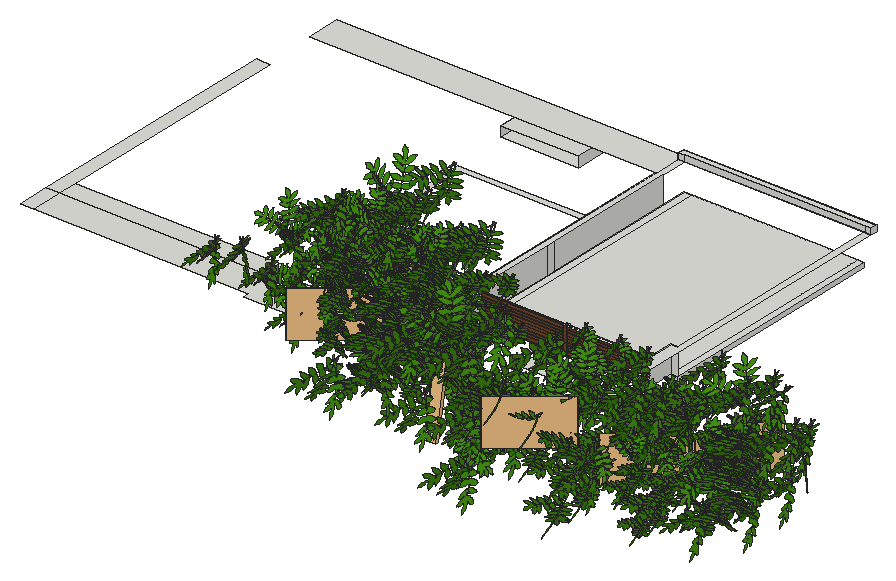
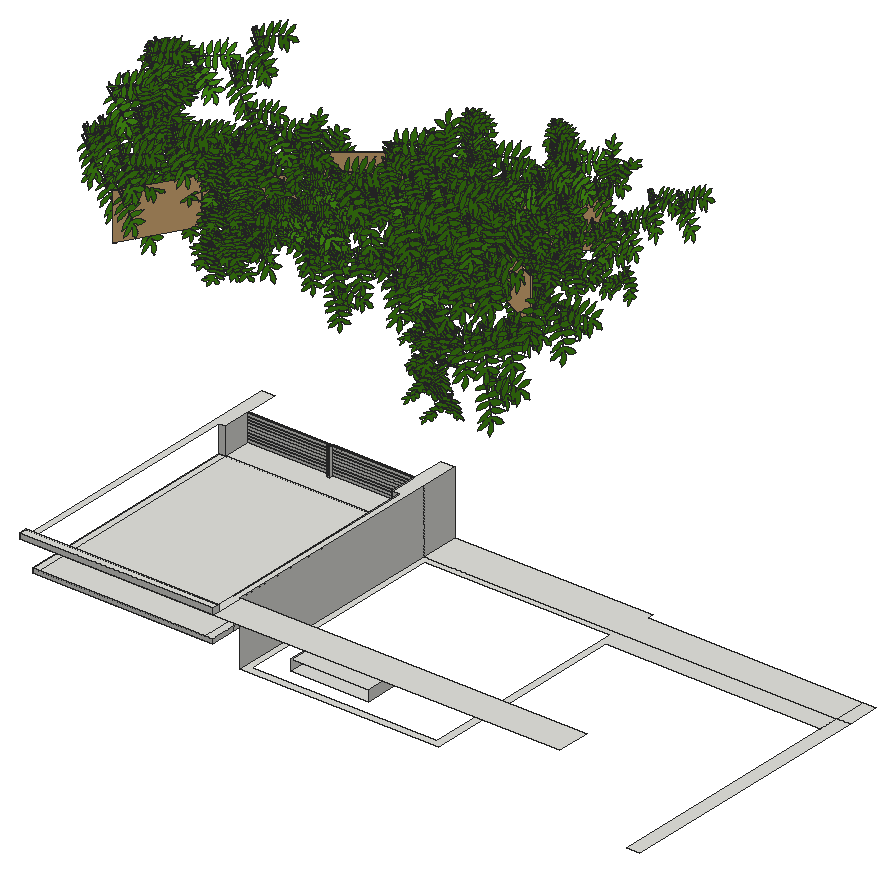
# SketchUp Ruby script. Lengths in inches.
U = 1.inch
M = Sketchup.active_model
def pt(a) = Geom::Point3d.new(a.map { |v| v * U })
def face(e, loops, mat)
  f = e.add_face(loops[0].map { |a| pt(a) })
  loops[1..].each { |l| e.add_face(l.map { |a| pt(a) }).erase! }
  f.material = f.back_material = mat if mat
  f
end
# faces: each face lists its corners as indices into pts; further lists are holes
def faces(e, pts, list, mat = nil) = list.each { |f| face(e, (f[0].is_a?(Array) ? f : [f]).map { |l| l.map { |i| pts[i] } }, mat) }
# xy, xz, yz: faces in a plane at the given z, y or x. An outline is a flat list of corners, or four numbers for a rectangle; further outlines are holes
def ring(l) = l.size == 4 ? [[l[0], l[1]], [l[2], l[1]], [l[2], l[3]], [l[0], l[3]]] : l.each_slice(2).to_a
def flat(e, list, mat, &to3) = list.each { |f| face(e, (f[0].is_a?(Array) ? f : [f]).map { |l| ring(l).map { |u, v| to3.(u, v) } }, mat) }
def xy(e, z, list, mat = nil) = flat(e, list, mat) { |x, y| [x, y, z] }
def xz(e, y, list, mat = nil) = flat(e, list, mat) { |x, z| [x, y, z] }
def yz(e, x, list, mat = nil) = flat(e, list, mat) { |y, z| [x, y, z] }
def lines(e, pts, list) = list.each { |a, b| e.add_line(pt(pts[a]), pt(pts[b])) }
# prism: a flat outline (further loops are holes) pulled along v
def prism(e, loops, v, mat = nil)
  f = face(e, loops, mat); d = Geom::Vector3d.new(v.map { |x| x * U })
  f.pushpull(f.normal.samedirection?(d) ? d.length : -d.length)
end
def box(e, o, s, mat = nil) = prism(e, [[o, [o[0] + s[0], o[1], o[2]], [o[0] + s[0], o[1] + s[1], o[2]], [o[0], o[1] + s[1], o[2]]]], [0, 0, s[2]], mat)
def at(x, y, z, deg = 0) = Geom::Transformation.translation(pt([x, y, z])) * Geom::Transformation.rotation(ORIGIN, Z_AXIS, deg.degrees)
def axes(o, x, y, z) = Geom::Transformation.new([*x, 0, *y, 0, *z, 0, *pt(o).to_a, 1])
def part(name) = M.definitions.add(name)
# library, detail: a bought-in or finely detailed component or shape, given as its bounding box
def library(name, o, s) = part(name).tap { |d| box(d.entities, o, s) }
def detail(e, o, s) = box(e.add_group.entities, o, s)
def put(e, d, t, mat = nil) = e.add_instance(d, t).tap { |i| i.material = mat if mat }
def group(e, t, mat = nil) = e.add_group.tap { |g| g.transformation = t; g.material = mat if mat }.entities
root = M.entities
M.materials.add("[Color D01]").color = [255, 242, 204]
M.materials.add("[Wood Veneer 01]").color = [120, 70, 37]
M.materials.add("hojas").color = [70, 150, 19]
c1 = part("rama-acacia")
p = [[-13.53,0.69,-1.07],[-13.38,0.86,-0.98],[-13.61,0.85,-1.06],[-14.07,0.85,-1.21],[-15.17,0.86,-1.58],[-15.95,0.92,-1.83],
  [-16.01,1,-1.83],[-16.01,1.17,-1.78],[-16.07,1.93,-1.6],[-16.4,2.73,-1.5],[-16.65,3.06,-1.5],[-17.13,4.01,-1.41],
  [-17.78,4.7,-1.44],[-18.28,5.07,-1.51],[-18.57,5.18,-1.58],[-18.91,5.47,-1.62],[-19.07,5.48,-1.67],[-19.35,5.61,-1.73],
  [-19.51,5.64,-1.78],[-19.38,5.57,-1.75],[-19.33,5.5,-1.75],[-19.31,5.23,-1.82],[-19.38,5.08,-1.89],[-19.41,4.84,-1.96],
  [-19.36,4.59,-2.01],[-19.43,4.55,-2.04],[-19.36,4.15,-2.125],[-19.21,3.7,-2.19],[-18.875,3.1,-2.24],[-18.61,2.78,-2.24],
  [-17.83,2.19,-2.13],[-17.4375,1.85,-2.09],[-17.04,1.49,-2.05],[-16.61,1.24,-1.97],[-16.17,1.0625,-1.87],[-16.06,0.95,-1.86],
  [-16.06,0.91,-1.87],[-16.32,0.9,-1.96],[-16.7,0.88,-2.1],[-17.05,0.91,-2.21],[-17.61,1.15,-2.33],[-18.06,1.29,-2.45],
  [-18.88,1.53,-2.67],[-20.25,1.46,-3.15],[-20.59,1.49,-3.26],[-20.79,1.37,-3.36],[-21.08,1.2,-3.5],[-21.28,1.22,-3.5625],
  [-21.48,0.94,-3.71],[-21.79,0.5,-3.93],[-22.02,0.17,-4.1],[-22.11,0.05,-4.16],[-22.21,-0.02,-4.21],[-22.375,-0.05,-4.28],
  [-22.375,-0.07,-4.28],[-22.18,-0.09,-4.22],[-22.11,-0.07,-4.19],[-21.78,-0.1,-4.09],[-21.6,-0.18,-4.05],[-21.52,-0.27,-4.04],
  [-21.33,-0.33,-4],[-20.94,-0.54,-3.92],[-20.6875,-0.63,-3.86],[-20.54,-0.68,-3.82],[-20.42,-0.67,-3.78],[-20.09,-0.46,-3.61],
  [-19.8,-0.24,-3.45],[-19.21,-0.02,-3.19],[-18.48,0.08,-2.92],[-17.72,0.38,-2.58],[-17.4,0.5,-2.4375],[-16.93,0.75,-2.21],
  [-16.78,0.8,-2.15],[-16.1,0.83,-1.91],[-16.0625,0.81,-1.9],[-16.08,0.77,-1.91],[-16.27,0.72,-1.99],[-16.88,0.39,-2.29],
  [-17.1875,0.15,-2.46],[-17.27,0.02,-2.52],[-17.94,-0.52,-2.89],[-17.94,-0.59,-2.91],[-18.08,-0.68,-2.99],[-18.13,-0.86,-3.05],
  [-18.56,-1.55,-3.38],[-18.71,-2.11,-3.58],[-18.79,-2.61,-3.74],[-18.86,-2.84,-3.83],[-18.87,-3.07,-3.89],[-18.84,-3.22,-3.92],
  [-18.8,-3.26,-3.92],[-18.76,-3.47,-3.96],[-18.76,-3.6,-4],[-18.67,-3.8,-4.02],[-18.61,-3.92,-4.04],[-18.58,-4.11,-4.07],
  [-18.53,-4.18,-4.08],[-18.58,-4.35,-4.14],[-18.65,-4.43,-4.18],[-18.72,-4.51,-4.23],[-18.8125,-4.51,-4.26],[-18.8125,-4.53,-4.26],
  [-18.72,-4.54,-4.24],[-18.66,-4.49,-4.21],[-18.58,-4.43,-4.16],[-18.35,-4.23,-4.03],[-18.32,-4.17,-4],[-18.22,-4.125,-3.95],
  [-18.1,-4,-3.88],[-17.79,-3.72,-3.7],[-17.68,-3.51,-3.61],[-17.32,-3.13,-3.38],[-17.24,-2.94,-3.31],[-16.78,-2.12,-2.93],
  [-16.48,-1.78,-2.73],[-16.3,-1.28,-2.54],[-16.05,-0.75,-2.3125],[-15.89,-0.2,-2.11],[-15.89,0.39,-1.95],[-15.96,0.79,-1.87],
  [-15.91,0.82,-1.84],[-15.27,0.8,-1.63],[-14.18,0.76,-1.27],[-13.78,0.73,-1.15],[-13.78,0.67,-1.16],[-14.23,0.54,-1.35],
  [-14.65,0.33,-1.55],[-14.97,0.02,-1.74],[-15.25,-0.36,-1.9375],[-15.57,-0.72,-2.14],[-15.96,-1.64,-2.52],[-16.2,-2.51,-2.84],
  [-16.2,-3.12,-3],[-16.14,-3.41,-3.06],[-16.1,-3.75,-3.14],[-16.1,-4.09,-3.23],[-16.2,-4.25,-3.3],[-16.2,-4.28,-3.3125],
  [-16.08,-4.19,-3.24],[-15.98,-4.08,-3.18],[-15.96,-3.94,-3.14],[-15.96,-3.8125,-3.1],[-15.9,-3.72,-3.06],[-15.68,-3.55,-2.9375],
  [-15.51,-3.49,-2.86],[-15.3,-3.33,-2.75],[-15.23,-3.17,-2.68],[-15.01,-3.03,-2.57],[-14.875,-2.83,-2.47],[-14.6,-2.59,-2.3125],
  [-14.4,-2.27,-2.16],[-14.12,-1.6,-1.89],[-13.91,-1.1,-1.68],[-13.67,-0.83,-1.53],[-13.53,-0.45,-1.38],[-13.53,0.67,-1.08],
  [-12.41,6.01,0.65],[-12.44,6.14,0.68],[-12.41,6.29,0.73],[-12.43,6.29,0.73],[-12.44,6.26,0.72],[-12.47,6.15,0.68],
  [-12.49,6.07,0.66],[-12.57,5.75,0.55],[-12.67,5.36,0.43],[-12.79,4.875,0.28],[-12.83,4.52,0.18],[-12.83,3.99,0.04],
  [-12.73,3.11,-0.18],[-12.58,2.52,-0.3125],[-12.3,1.97,-0.41],[-11.88,1.51,-0.46],[-11.37,1.0625,-0.48],[-10.75,0.75,-0.45],
  [-10.75,0.68,-0.47],[-12.55,0.7,-0.79],[-13.21,0.79,-0.89],[-13.2,0.67,-0.92],[-12.56,0.62,-0.82],[-11.15,0.56,-0.58],
  [-10.79,0.54,-0.52],[-10.72,0.52,-0.51],[-10.72,0.5,-0.52],[-10.87,0.47,-0.55],[-11.14,0.41,-0.62],[-11.39,0.27,-0.7],
  [-11.625,-0.01,-0.82],[-11.8,-0.43,-0.96],[-11.83,-0.57,-1],[-12.02,-1.08,-1.17],[-12.1,-1.39,-1.27],[-12.17,-1.95,-1.4375],
  [-12.17,-2.77,-1.65],[-12.09,-3.59,-1.86],[-11.86,-4.26,-2],[-11.8125,-4.4,-2.03],[-11.84,-4.49,-2.05],[-11.91,-4.6,-2.1],
  [-11.97,-4.65,-2.12],[-11.98,-4.67,-2.13],[-11.92,-4.65,-2.11],[-11.84,-4.59,-2.08],[-11.77,-4.52,-2.05],[-11.74,-4.47,-2.03],
  [-11.37,-4.3125,-1.92],[-10.95,-4.0625,-1.78],[-10.82,-3.89,-1.71],[-10.64,-3.57,-1.59],[-10.41,-3.05,-1.41],[-10.27,-2.73,-1.3],
  [-10.07,-1.88,-1.03],[-10.15,-0.71,-0.73],[-10.31,-0.1,-0.6],[-10.5,0.4,-0.5],[-10.5,0.48,-0.48],[-10.44,0.53,-0.45],
  [-10.39,0.64,-0.42],[-10.52,0.73,-0.42],[-10.44,0.93,-0.35],[-10.44,1.2,-0.28],[-10.32,1.47,-0.18],[-10.48,2.6875,0.12],
  [-10.43,2.96,0.2],[-10.75,3.87,0.38],[-11.26,4.93,0.57],[-11.8,5.54,0.64],[-12.37,5.93,0.64],[-7.78,0.19,-0.06],
  [-7.78,0.25,-0.04],[-7.75,0.39,0],[-7.89,0.4,-0.02],[-7.96,0.46,-0.02],[-7.96,0.49,-0.01],[-7.76,0.62,0.06],
  [-7.53,0.99,0.2],[-7.31,1.78,0.45],[-7.31,2.74,0.71],[-7.63,3.6875,0.9],[-8.02,4.57,1.07],[-8.66,5.23,1.13],
  [-8.83,5.4,1.14],[-8.92,5.54,1.16],[-9.1,5.64,1.16],[-9.08,5.6,1.15],[-9.02,5.56,1.15],[-8.94,5.46,1.14],
  [-8.9,5.37,1.12],[-8.9375,5.25,1.08],[-9.14,4.92,0.96],[-9.31,4.5625,0.83],[-9.39,3.73,0.6],[-9.44,2.76,0.32],
  [-9.23,1.59,0.05],[-8.82,0.9,-0.06],[-8.36,0.59,-0.0625],[-8.14,0.51,-0.04],[-8.05,0.48,-0.03],[-8.05,0.46,-0.04],
  [-8.12,0.43,-0.06],[-10.1,0.49,-0.4],[-8.22,0.3125,-0.11],[-8.22,0.25,-0.125],[-8.53,0.13,-0.21],[-8.8,-0.16,-0.34],
  [-8.96,-0.61,-0.49],[-8.96,-0.87,-0.56],[-9.16,-1.42,-0.74],[-9.13,-1.77,-0.83],[-9.09,-1.83,-0.84],[-9.125,-1.92,-0.87],
  [-9.125,-2.13,-0.93],[-9.08,-2.23,-0.95],[-9.15,-2.39,-1],[-9.11,-2.67,-1.07],[-9.03,-2.86,-1.11],[-9.07,-3.03,-1.16],
  [-8.97,-3.23,-1.19],[-8.93,-3.44,-1.24],[-8.93,-3.71,-1.32],[-8.79,-4.05,-1.38],[-8.7,-4.25,-1.42],[-8.7,-4.39,-1.46],
  [-8.76,-4.53,-1.5],[-8.77,-4.65,-1.54],[-8.64,-4.55,-1.49],[-8.27,-4.22,-1.33],[-8.1875,-4.06,-1.27],[-8.07,-3.98,-1.23],
  [-7.98,-3.79,-1.17],[-7.79,-3.59,-1.08],[-7.64,-3.3,-0.97],[-7.64,-3.25,-0.96],[-7.59,-3.21,-0.9375],[-7.52,-2.93,-0.85],
  [-7.52,-2.85,-0.83],[-7.47,-2.81,-0.81],[-7.3,-2.09,-0.59],[-7.32,-2.01,-0.57],[-7.27,-1.95,-0.54],[-7.1875,-1.57,-0.42],
  [-7.17,-1.46,-0.39],[-7.17,-1.16,-0.3125],[-7.23,-0.61,-0.17],[-7.49,-0.15,-0.1],[-13.39,-0.07,-1.23],[-13.39,0.25,-1.14],
  [-13.49,0.5625,-1.09],[-13.8,1.01,-1.08],[-13.61,0.91,-1.04],[-13.38,0.92,-0.96],[-13.32,1.03,-0.91],[-13.32,1.35,-0.82],
  [-13.28,1.49,-0.77],[-13.28,1.99,-0.64],[-13.44,2.67,-0.51],[-13.72,3.31,-0.43],[-13.93,3.71,-0.4],[-14.1,4.39,-0.27],
  [-14.5625,5.06,-0.25],[-14.89,5.62,-0.21],[-15.33,6.1,-0.23],[-15.65,6.8,-0.15],[-15.79,6.89,-0.18],[-15.61,6.52,-0.22],
  [-15.51,6.32,-0.24],[-15.45,6.28,-0.23],[-15.52,6,-0.32],[-15.63,5.6875,-0.45],[-15.77,4.97,-0.68],[-15.7,4.25,-0.85],
  [-15.46,3,-1.11],[-15,2.03,-1.21],[-14.3,1.29,-1.17],[-4.5625,0.33,0.09],[-4.22,0.49,0.13],[-4,0.7,0.1875],
  [-3.86,0.99,0.26],[-3.77,1.41,0.38],[-3.7,1.73,0.46],[-3.77,1.99,0.53],[-3.85,2.17,0.58],[-3.88,2.57,0.6875],
  [-3.98,2.9,0.78],[-4.0625,2.97,0.8],[-4.1,3.14,0.84],[-4.1875,3.25,0.87],[-4.27,3.55,0.95],[-4.31,3.71,0.99],
  [-4.42,3.9,1.04],[-4.625,4.2,1.125],[-4.72,4.39,1.18],[-4.89,4.57,1.23],[-4.98,4.73,1.27],[-5,4.72,1.26],
  [-5.01,4.51,1.21],[-4.96,4.32,1.16],[-4.97,4.27,1.14],[-5.14,3.78,1.01],[-5.3,3.39,0.91],[-5.44,2.76,0.74],
  [-5.5,2.09,0.56],[-5.57,1.78,0.48],[-5.57,1.42,0.38],[-5.57,1.09,0.29],[-5.47,0.72,0.19],[-5.22,0.44,0.12],
  [-4.93,0.27,0.07],[-4.76,0.22,0.06],[-4.76,0.18,0.05],[-4.83,0.16,0.04],[-5.26,0,0],[-5.34,-0.04,-0.01],
  [-5.47,-0.22,-0.06],[-5.51,-0.6,-0.16],[-5.42,-1.09,-0.29],[-5.28,-1.49,-0.4],[-5.21,-1.87,-0.5],[-5.11,-2.15,-0.57],
  [-5.08,-2.34,-0.63],[-5.01,-2.47,-0.66],[-4.96,-2.69,-0.72],[-4.86,-2.9375,-0.79],[-4.84,-3.07,-0.82],[-4.77,-3.18,-0.85],
  [-4.74,-3.43,-0.92],[-4.7,-3.71,-0.99],[-4.62,-3.89,-1.04],[-4.58,-3.98,-1.07],[-4.58,-3.83,-1.03],[-4.51,-3.67,-0.98],
  [-4.3,-3.32,-0.89],[-4.16,-3.09,-0.83],[-4.16,-2.98,-0.8],[-4.11,-2.92,-0.78],[-4.02,-2.8,-0.75],[-3.95,-2.59,-0.69],
  [-3.95,-2.33,-0.625],[-3.86,-2.26,-0.6],[-3.86,-2.02,-0.54],[-3.86,-1.44,-0.39],[-3.94,-1.22,-0.33],[-3.94,-1.08,-0.29],
  [-4,-0.96,-0.26],[-4,-0.87,-0.23],[-4.0625,-0.8125,-0.22],[-4.16,-0.54,-0.14],[-4.39,-0.24,-0.06],[-4.61,-0.08,-0.02],
  [-4.77,-0.03,-0.01],[-4.77,-0.01,0],[-4.65,-0.01,0],[-4.61,0.19,0.05],[-4.66,0.23,0.0625],[-4.63,0.29,0.08],
  [-4.07,0.17,0.04],[0,-0.24,-0.06],[0,0,0],[-0.5,0.04,0.01],[-1.58,0.08,0.02],[-13.78,0.67,-1.08]]
faces(c1.entities,p,[[0,1,2,3,4,5,6,7,8,9,10,11,12,13,14,15,16,17,18,19,20,21,22,23,24,25,26,27,28,29,30,31,32,33,34,35,36,37,38,39,40,41,42,43,44,45,46,47,48,49,50,51,52,53,54,55,56,57,58,59,60,61,62,63,64,65,66,67,68,69,70,71,72,73,74,75,76,77,78,79,80,81,82,83,84,85,86,87,88,89,90,91,92,93,94,95,96,97,98,99,100,101,102,103,104,105,106,107,108,109,110,111,112,113,114,115,116,117,118,119,120,121,122,123,124,125,126,127,128,129,130,131,132,133,134,135,136,137,138,139,140,141,142,143,144,145,146,147,148,149,150,151,152,153,154,155],[156,157,158,159,160,161,162,163,164,165,166,167,168,169,170,171,172,173,174,175,176,177,178,179,180,181,182,183,184,185,186,187,188,189,190,191,192,193,194,195,196,197,198,199,200,201,202,203,204,205,206,207,208,209,210,211,212,213,214,215,216,217,218,219,220,221,222,223,224,225,226],[227,228,229,230,231,232,233,234,235,236,237,238,239,240,241,242,243,244,245,246,247,248,249,250,251,252,253,254,255,256,257,258,216,215,259,260,261,262,263,264,265,266,267,268,269,270,271,272,273,274,275,276,277,278,279,280,281,282,283,284,285,286,287,288,289,290,291,292,293,294,295,296,297,298,299,300,301,302,303],[154,304,305,306,155],[307,308,1,309,310,311,312,313,314,315,316,317,318,319,320,321,322,323,324,325,326,327,328,329,330,331,332],[333,334,335,336,337,338,339,340,341,342,343,344,345,346,347,348,349,350,351,352,353,354,355,356,357,358,359,360,361,362,363,364,365,366,367,368,369,370,371,372,373,374,375,376,377,378,379,380,381,382,383,384,385,386,387,388,389,390,391,392,393,394,395,396,397,398,399,400,401,402,403,404,405,406,407,408,409,410,411,412,413],[0,177,1],[308,2,1],
  [176,1,177],[414,411,410,415,416,417,418],[228,370,229],[369,229,370]],"hojas")
lines(c1.entities,p,[[155,419]])
c2 = part("Group\#83")
put(c2.entities,c1,axes([10.13,10.27,0],[0.45315,0.21131,0],[-0.21131,0.45315,0],[0,0,0.5]))
put(c2.entities,c1,axes([10.13,10.27,0],[0.11638,0.47539,0.10227],[-0.48087,0.12813,-0.0484],[-0.07223,-0.08709,0.48703]))
put(c2.entities,c1,axes([9.58,10.26,-0.7],[0.1449,0.38901,-0.2787],[-0.10883,0.31035,0.37662],[0.46601,-0.04848,0.17461]))
c3 = part("Group\#84")
put(c3.entities,c2,axes([24.99,4.24,9.59],[0.78856,0.61496,0],[0.01473,-0.01889,0.99971],[0.61478,-0.78833,-0.02396]))
put(c3.entities,c2,axes([39.5,6.625,12.55],[0.6544,0.49291,0.57341],[-0.44023,-0.3682,0.81892],[0.61478,-0.78833,-0.02396]))
put(c3.entities,c2,axes([32.34,3.7,6.88],[0.78856,0.61496,0],[0.01473,-0.01889,0.99971],[0.61478,-0.78833,-0.02396]))
put(c3.entities,c2,axes([43.14,6.65,17.54],[0.78856,0.61496,0],[0.35273,-0.4523,0.81915],[0.50374,-0.64595,-0.57358]))
put(c3.entities,c2,axes([12.2,6.2,16.68],[0.7209,0.54936,0.4225],[-0.31991,-0.27701,0.90605],[0.61478,-0.78833,-0.02396]))
put(c3.entities,c2,axes([49.9375,3.79,26.09],[0.78856,0.61496,0],[0.01473,-0.01889,0.99971],[0.61478,-0.78833,-0.02396]))
put(c3.entities,c2,axes([36.11,4.9375,33.94],[0.78856,0.61496,0],[0.01473,-0.01889,0.99971],[0.61478,-0.78833,-0.02396]))
put(c3.entities,c2,axes([39.61,3.79,23.47],[0.78856,0.61496,0],[0.01473,-0.01889,0.99971],[0.61478,-0.78833,-0.02396]))
put(c3.entities,c2,axes([25.59,6.5625,46.47],[-0.40704,-0.29112,-0.86578],[0.67555,0.54201,-0.49986],[0.61478,-0.78833,-0.02396]))
put(c3.entities,c2,axes([54.97,1.98,11.65],[0.78856,0.61496,0],[0.01473,-0.01889,0.99971],[0.61478,-0.78833,-0.02396]))
put(c3.entities,c2,axes([32.97,3.79,19.14],[0.78856,0.61496,0],[0.01473,-0.01889,0.99971],[0.61478,-0.78833,-0.02396]))
put(c3.entities,c2,axes([24.24,3.79,21.99],[0.78856,0.61496,0],[0.01473,-0.01889,0.99971],[0.61478,-0.78833,-0.02396]))
put(c3.entities,c2,axes([16.86,4.24,12.3],[0.78856,0.61496,0],[0.01473,-0.01889,0.99971],[0.61478,-0.78833,-0.02396]))
put(c3.entities,c2,axes([1.23,3.9375,19.07],[0.78856,0.61496,0],[0.01473,-0.01889,0.99971],[0.61478,-0.78833,-0.02396]))
put(c3.entities,c2,axes([29.05,5.25,29.11],[0.78856,0.61496,0],[0.21033,-0.2697,0.93969],[0.57787,-0.741,-0.34202]))
put(c3.entities,c2,axes([24.16,3.79,-0.1],[0.78856,0.61496,0],[0.01473,-0.01889,0.99971],[0.61478,-0.78833,-0.02396]))
c4 = library("Group\#86",[0,0,0],[9.94,2.45,66.78])
c5 = library("Group\#85",[0,0,0],[130.24,0.88,39.6])
xy(root,272.11,[[537.75,397.34,536.96,397.45,536.22,397.75,535.59,398.24,535.1,398.875,534.79,399.61,534.6875,400.4,534.79,401.2,535.1,401.9375,535.59,402.57,536.22,403.06,536.96,403.36,537.75,403.47,538.54,403.36,539.28,403.06,539.92,402.57,540.4,401.9375,540.71,401.2,540.8125,400.4,540.71,399.61,540.4,398.875,539.92,398.24,539.28,397.75,538.54,397.45],[638.61,397.34,637.82,397.45,637.08,397.75,636.44,398.24,635.96,398.875,635.65,399.61,635.55,400.4,635.65,401.2,635.96,401.9375,636.44,402.57,637.08,403.06,637.82,403.36,638.61,403.47,639.4,403.36,640.14,403.06,640.77,402.57,641.26,401.9375,641.57,401.2,641.67,400.4,641.57,399.61,641.26,398.875,640.77,398.24,640.14,397.75,639.4,397.45]])
xy(root,287.5625,[[400.76,389.67,660.05,389.67,660.05,440.22,118.89,440.22,118.89,397.92,400.76,397.92],[101.6875,397.92,118.89,440.22],[101.6875,440.22,118.89,784.05],[[118.89,440.22,660.05,440.22,660.05,739.86,400.76,739.86,400.76,466.49,118.89,466.49],[408.8,448.26,652.01,731.82]]])
xy(root,302.375,[[726.09,431.86,726.09,469.66,842.22,469.66,842.22,434.99,837.78,434.99,837.78,431.86,836.22,431.86,836.22,434.99,831.78,434.99,831.78,431.86,830.34,431.86,830.34,434.99,825.9,434.99,825.9,431.86,824.34,431.86,824.34,434.99,819.9,434.99,819.9,431.86,818.34,431.86,818.34,434.99,813.9,434.99,813.9,431.86,812.34,431.86,812.34,434.99,807.9,434.99,807.9,431.86],[807.9,431.86,812.34,434.99],[813.9,431.86,818.34,434.99],[819.9,431.86,824.34,434.99],[825.9,431.86,830.34,434.99],
  [831.78,431.86,836.22,434.99],[837.78,431.86,842.22,434.99]])
xy(root,329.3125,[[668.6,469.66,678.11,774.73]])
xy(root,329.3125,[[678.11,469.66,903.88,774.73]],"[Color D01]")
xy(root,335.3125,[[678.11,431.86,784.78,431.86,784.78,437.8,788.85,437.8,788.85,431.86,895.55,431.86,895.55,469.66,678.11,469.66],[784.78,431.86,788.85,437.8],[668.6,469.66,678.11,774.73],[678.11,469.66,895.55,774.73],[895.55,469.66,903.88,774.73]])
xy(root,340.08,[[456.09,739.86,558.27,784.05]])
xy(root,353.76,[[456.09,739.86,558.27,784.05]])
xy(root,370.4375,[[660.05,389.67,678.11,389.67,678.11,469.66,668.6,469.66,668.6,775.49,660.05,775.6875],[895.55,389.67,912.4375,389.67,912.4375,775.49,903.88,775.49,903.88,469.66,895.55,469.66],[678.11,431.86,784.78,434.99],[784.78,431.86,788.85,434.99],[788.85,431.86,895.55,434.99],
  [784.78,434.99,788.85,437.8],[207.07,739.86,660.05,784.05],[668.6,775.49,660.05,775.6875,660.05,784.05,912.4375,784.05,912.4375,775.49]])
xy(root,378,[[668.6,775.49,912.4375,775.49,912.4375,784.05,660.05,784.05,660.05,775.6875]])
xz(root,431.86,[[784.78,335.3125,788.85,370.4375],[678.11,337.3125,784.78,340.4375],[788.85,337.3125,895.55,340.4375],[678.11,341.0625,784.78,344.1875],[788.85,341.0625,895.55,344.1875],
  [678.11,344.8125,784.78,347.9375],[788.85,344.8125,895.55,347.9375],[678.11,348.5625,784.78,351.6875],[788.85,348.5625,895.55,351.6875],[678.11,352.3125,784.78,355.4375],
  [788.85,352.3125,895.55,355.4375],[678.11,356.0625,784.78,359.1875],[788.85,356.0625,895.55,359.1875],[678.11,359.8125,784.78,362.9375],[788.85,359.8125,895.55,362.9375],
  [678.11,363.5625,784.78,366.6875],[788.85,363.5625,895.55,366.6875],[678.11,367.3125,784.78,370.4375],[788.85,367.3125,895.55,370.4375]],"[Wood Veneer 01]")
xz(root,434.99,[[678.11,337.3125,895.55,340.4375],[678.11,341.0625,895.55,344.1875],[678.11,344.8125,895.55,347.9375],[678.11,348.5625,895.55,351.6875],[678.11,352.3125,895.55,355.4375],
  [678.11,356.0625,895.55,359.1875],[678.11,359.8125,895.55,362.9375],[678.11,363.5625,895.55,366.6875],[678.11,367.3125,895.55,370.4375]])
xz(root,437.8,[[784.78,335.3125,786.83,370.4375],[786.83,335.3125,788.85,370.4375]])
xz(root,469.66,[[668.6,329.3125,903.88,335.3125],[668.6,335.3125,678.11,370.4375],[895.55,335.3125,903.88,370.4375]])
xz(root,774.73,[[668.6,329.3125,903.88,335.3125]])
xz(root,775.49,[[668.6,370.4375,903.88,378],[903.88,370.4375,912.4375,378]])
xz(root,784.05,[[660.05,370.4375,912.4375,378]])
yz(root,456.09,[[739.86,340.08,784.05,353.76]])
yz(root,558.27,[[739.86,340.08,784.05,353.76]])
yz(root,660.05,[[389.67,287.5625,440.22,370.4375],[440.22,287.5625,739.86,370.4375],[775.6875,370.4375,784.05,378]])
yz(root,668.6,[[469.66,329.3125,551.1875,335.3125],[551.1875,329.3125,562.07,335.3125],[562.07,329.3125,739.86,335.3125],[739.86,329.3125,774.73,335.3125],[469.66,335.3125,551.1875,370.4375],
  [551.1875,335.3125,562.07,370.4375],[562.07,335.3125,739.86,370.4375]])
yz(root,678.11,[[431.86,335.3125,469.66,335.3125,469.66,370.4375,434.99,370.4375,434.99,367.3125,431.86,367.3125,431.86,366.6875,434.99,366.6875,434.99,363.5625,431.86,363.5625,431.86,362.9375,434.99,362.9375,434.99,359.8125,431.86,359.8125,431.86,359.1875,434.99,359.1875,434.99,356.0625,431.86,356.0625,431.86,355.4375,434.99,355.4375,434.99,352.3125,431.86,352.3125,431.86,351.6875,434.99,351.6875,434.99,348.5625,431.86,348.5625,431.86,347.9375,434.99,347.9375,434.99,344.8125,431.86,344.8125,431.86,344.1875,434.99,344.1875,434.99,341.0625,431.86,341.0625,431.86,340.4375,434.99,340.4375,434.99,337.3125,431.86,337.3125]])
yz(root,784.78,[[431.86,335.3125,437.8,370.4375]])
yz(root,788.85,[[431.86,335.3125,437.8,370.4375]])
yz(root,895.55,[[431.86,335.3125,431.86,337.3125,434.99,337.3125,434.99,340.4375,431.86,340.4375,431.86,341.0625,434.99,341.0625,434.99,344.1875,431.86,344.1875,431.86,344.8125,434.99,344.8125,434.99,347.9375,431.86,347.9375,431.86,348.5625,434.99,348.5625,434.99,351.6875,431.86,351.6875,431.86,352.3125,434.99,352.3125,434.99,355.4375,431.86,355.4375,431.86,356.0625,434.99,356.0625,434.99,359.1875,431.86,359.1875,431.86,359.8125,434.99,359.8125,434.99,362.9375,431.86,362.9375,431.86,363.5625,434.99,363.5625,434.99,366.6875,431.86,366.6875,431.86,367.3125,434.99,367.3125,434.99,370.4375,469.66,370.4375,469.66,335.3125],[431.86,337.3125,434.99,340.4375],[431.86,341.0625,434.99,344.1875],[431.86,344.8125,434.99,347.9375],[431.86,348.5625,434.99,351.6875],
  [431.86,352.3125,434.99,355.4375],[431.86,356.0625,434.99,359.1875],[431.86,359.8125,434.99,362.9375],[431.86,363.5625,434.99,366.6875],[431.86,367.3125,434.99,370.4375]])
yz(root,903.88,[[469.66,329.3125,774.73,335.3125]])
yz(root,912.4375,[[775.49,370.4375,784.05,378]])
p = [[660.05,775.6875,370.4375],[668.6,775.49,370.4375],[668.6,775.49,378],[660.05,775.6875,378],[786.83,437.8,335.3125],[786.83,437.86,335.3125]]
faces(root,p,[[0,1,2,3]])
lines(root,p,[[4,5]])
put(root,c3,axes([958.28,157.5625,300.52],[-3.24317,2.72134,0],[-2.72134,-3.24317,0],[0,0,4.23366]))
put(root,c3,axes([862.99,121.8,318.99],[4.332,0,0],[0,4.332,0],[0,0,4.332]))
put(root,c2,axes([881.26,84.79,327.97],[1.23016,5.76213,0],[0.13804,-0.02947,5.89028],[5.76047,-1.2298,-0.14116]))
put(root,c3,axes([577.77,218.28,350.75],[4.15786,0,0],[0,6.02589,0],[0,0,6.02589]))
put(root,c3,axes([1022.02,125.42,352.375],[2.888,0,0],[0,2.888,0],[0,0,2.888]))
put(root,c3,axes([935.56,71.31,364.45],[3.91235,1.82436,0],[-1.82436,3.91235,0],[0,0,4.3168]))
put(root,c2,axes([1199.375,164.33,367.26],[0.56308,6.22693,0],[0.13677,-0.10234,4.56538],[5.70745,-4.27056,-0.10941]))
put(root,c2,axes([918.52,115.35,369.13],[1.23016,5.76213,0],[0.13804,-0.02947,5.89028],[5.76047,-1.2298,-0.14116]))
put(root,c3,axes([1016.9,183.76,369.26],[3.3592,0,0],[0,3.3592,0],[0,0,3.3592]))
put(root,c3,axes([999.52,292.13,372.66],[1.3756,-2.38261,0],[4.40783,2.54486,0],[0,0,2.7512]))
put(root,c2,axes([883.33,90,385.1],[1.23016,5.76213,0],[0.13804,-0.02947,5.89028],[5.76047,-1.2298,-0.14116]))
put(root,c4,axes([836.13,139.52,381.99],[1.51495,0.09294,0.08178],[-0.06642,1.45755,-0.42607],[-0.10447,0.42108,1.45677]))
put(root,c2,axes([1194.2,83.55,390.29],[0.56308,6.22693,0],[0.13677,-0.10234,4.56538],[5.70745,-4.27056,-0.10941]))
put(root,c2,axes([1027.19,193.35,397.22],[1.23016,5.76213,0],[0.13804,-0.02947,5.89028],[5.76047,-1.2298,-0.14116]))
put(root,c2,axes([939.78,155.71,402.55],[1.08687,4.70315,3.37853],[-0.59251,-3.32916,4.82504],[5.76047,-1.2298,-0.14116]))
put(root,c2,axes([1232.09,182.35,399.16],[0.56308,6.22693,0],[0.13677,-0.10234,4.56538],[5.70745,-4.27056,-0.10941]))
put(root,c2,axes([846.6,59.18,401.03],[1.23016,5.76213,0],[0.13804,-0.02947,5.89028],[5.76047,-1.2298,-0.14116]))
put(root,c2,axes([956.1,169.6,431.92],[1.23016,5.76213,0],[3.30502,-0.70559,4.82642],[4.72006,-1.00769,-3.3795]))
put(root,c3,axes([698.75,124.16,403.51],[3.5264,0,0],[0,3.5264,0],[0,0,3.5264]))
put(root,c3,axes([950.48,112.81,405.82],[1.14986,2.46588,0],[-2.46588,1.14986,0],[0,0,2.7208]))
put(root,c5,axes([1185.97,290.1,404.73],[-0.38869,-0.65309,0],[0.26123,-0.15547,0],[0,0,1.52]))
put(root,c5,axes([1058.77,146.67,404.73],[0.59528,0.47249,0],[-0.189,0.23811,0],[0,0,1.52]))
put(root,c2,axes([1200.81,169.49,411.54],[0.56308,6.22693,0],[0.13677,-0.10234,4.56538],[5.70745,-4.27056,-0.10941]))
put(root,c2,axes([818.18,50.39,426.85],[1.17324,5.2098,2.48934],[-0.39478,-2.46189,5.33841],[5.76047,-1.2298,-0.14116]))
put(root,c2,axes([1248.27,219.78,425.0625],[0.5397,5.0421,2.61859],[-0.21093,-3.65545,3.73974],[5.70745,-4.27056,-0.10941]))
put(root,c2,axes([1168.63,150.91,423.89],[0.56308,6.22693,0],[0.13677,-0.10234,4.56538],[5.70745,-4.27056,-0.10941]))
put(root,c3,axes([1155.53,200.63,423.29],[1.3756,-2.38261,0],[4.40783,2.54486,0],[0,0,2.7512]))
put(root,c3,axes([698.72,200.63,423.29],[1.3756,-2.38261,0],[4.40783,2.54486,0],[0,0,2.7512]))
put(root,c3,axes([698.72,203.79,423.29],[1.3756,-2.38261,0],[4.40783,2.54486,0],[0,0,2.7512]))
put(root,c3,axes([756.51,332.32,425.6],[-2.32535,-2.77124,0],[2.77124,-2.32535,0],[0,0,3.6176]))
put(root,c2,axes([1167.4,234.37,427.91],[0.56308,6.22693,0],[0.13677,-0.10234,4.56538],[5.70745,-4.27056,-0.10941]))
put(root,c3,axes([771.92,151.45,434.04],[1.52,0,0],[0,1.52,0],[0,0,1.52]))
put(root,c2,axes([777.24,-1.37,440.92],[1.23016,5.76213,0],[0.13804,-0.02947,5.89028],[5.76047,-1.2298,-0.14116]))
put(root,c2,axes([921.03,118.15,441.35],[1.23016,5.76213,0],[0.13804,-0.02947,5.89028],[5.76047,-1.2298,-0.14116]))
put(root,c2,axes([1142.08,154.375,443.9],[0.56813,5.60027,1.92941],[-0.11401,-2.72437,4.13764],[5.70745,-4.27056,-0.10941]))
put(root,c2,axes([974.37,97.2,442.73],[2.99653,2.33684,0],[0.05598,-0.07179,3.79891],[2.33617,-2.99567,-0.09104]))
put(root,c2,axes([1023.89,86.27,443.58],[3.90962,0.89903,-0.09577],[0.09521,0.01329,4.01165],[0.89909,-3.91077,-0.00838]))
put(root,c2,axes([1095.03,68.98,443.21],[-0.55492,3.97424,0],[0.09521,0.01329,4.01165],[3.9731,0.55477,-0.09614]))
put(root,c2,axes([1136.01,118.75,443.21],[-0.55492,3.97424,0],[0.09521,0.01329,4.01165],[3.9731,0.55477,-0.09614]))
put(root,c5,axes([956.61,82.95,439.89],[0.59528,0.47249,0],[-0.189,0.23811,0],[0,0,1.52]))
put(root,c3,axes([705.62,173.56,446.58],[3.3592,0,0],[0,3.3592,0],[0,0,3.3592]))
put(root,c3,axes([606.44,195.9,446.58],[3.3592,0,0],[0,3.3592,0],[0,0,3.3592]))
put(root,c2,axes([1241.87,199.875,449.9375],[0.56308,6.22693,0],[0.13677,-0.10234,4.56538],[5.70745,-4.27056,-0.10941]))
put(root,c3,axes([697.6,136.43,450.68],[1.52,0,0],[0,1.52,0],[0,0,1.52]))
put(root,c2,axes([1108.1,113.04,454.81],[0.56308,6.22693,0],[0.13677,-0.10234,4.56538],[5.70745,-4.27056,-0.10941]))
put(root,c2,axes([1234.22,184.44,455.14],[0.56308,6.22693,0],[0.13677,-0.10234,4.56538],[5.70745,-4.27056,-0.10941]))
put(root,c2,axes([881.65,85.11,458.15],[1.23016,5.76213,0],[0.13804,-0.02947,5.89028],[5.76047,-1.2298,-0.14116]))
put(root,c3,axes([623.82,5.625,456.34],[3.03807,2.12728,0],[-4.25456,6.07614,0],[0,0,3.7088]))
put(root,c3,axes([684.53,265.61,455.46],[1.3756,-2.38261,0],[4.40783,2.54486,0],[0,0,2.7512]))
put(root,c2,axes([1198.97,59.72,482.22],[0.56308,6.22693,0],[3.2746,-2.4502,3.74081],[4.67661,-3.49924,-2.61934]))
put(root,c2,axes([951,143.3,466.85],[1.23016,5.76213,0],[0.13804,-0.02947,5.89028],[5.76047,-1.2298,-0.14116]))
put(root,c2,axes([1167.4,234.37,466.17],[0.56308,6.22693,0],[0.13677,-0.10234,4.56538],[5.70745,-4.27056,-0.10941]))
put(root,c2,axes([1199.71,164.51,468.16],[0.56308,6.22693,0],[0.13677,-0.10234,4.56538],[5.70745,-4.27056,-0.10941]))
put(root,c2,axes([945.72,74.71,470.77],[2.99653,2.33684,0],[0.05598,-0.07179,3.79891],[2.33617,-2.99567,-0.09104]))
put(root,c3,axes([752.66,214.39,470.24],[1.74367,-2.49022,0],[2.49022,1.74367,0],[0,0,3.04]))
put(root,c3,axes([662.91,168.05,470.24],[1.95407,-2.32878,0],[2.32878,1.95407,0],[0,0,3.04]))
put(root,c2,axes([1247.17,129.42,474.9],[0.56308,6.22693,0],[0.13677,-0.10234,4.56538],[5.70745,-4.27056,-0.10941]))
put(root,c2,axes([839.68,44.25,481.17],[1.23016,5.76213,0],[0.13804,-0.02947,5.89028],[5.76047,-1.2298,-0.14116]))
put(root,c5,axes([663.78,258.38,475.54],[1.35959,-0.67964,0],[0.67964,1.35959,0],[0,0,1.52]))
put(root,c5,axes([699.66,83.92,476.41],[0.59528,0.47249,0],[-0.189,0.23811,0],[0,0,1.52]))
put(root,c2,axes([918.99,66.17,482.09],[3.79458,0.19598,-0.05222],[0.05598,-0.07179,3.79891],[0.19494,-3.79426,-0.07457]))
put(root,c2,axes([897.8,109.88,500.1],[1.23016,5.76213,0],[1.97076,-0.42074,5.53665],[5.41463,-1.15597,-2.01517]))
put(root,c2,axes([1124.07,202.45,486.88],[0.56308,6.22693,0],[0.13677,-0.10234,4.56538],[5.70745,-4.27056,-0.10941]))
put(root,c2,axes([1212.65,185.99,500.67],[0.56308,6.22693,0],[1.95262,-1.46104,4.29128],[5.36478,-4.01417,-1.5619]))
put(root,c2,axes([877.24,102.74,602.41],[-0.73463,-2.85554,-5.10114],[0.99633,5.00488,-2.94514],[5.76047,-1.2298,-0.14116]))
put(root,c2,axes([1193.53,187.5625,579.97],[-0.39999,-3.02484,-3.95373],[0.41926,5.44385,-2.28269],[5.70745,-4.27056,-0.10941]))
put(root,c2,axes([1141.37,83.96,507.99],[0.56308,6.22693,0],[0.13677,-0.10234,4.56538],[5.70745,-4.27056,-0.10941]))
put(root,c3,axes([703.45,160.16,505.97],[1.16439,-0.97704,0],[0.97704,1.16439,0],[0,0,1.52]))
put(root,c2,axes([1217.35,127.28,521.29],[0.56308,6.22693,0],[0.13677,-0.10234,4.56538],[5.70745,-4.27056,-0.10941]))
put(root,c2,axes([1141.58,48.66,532.37],[0.56308,6.22693,0],[0.13677,-0.10234,4.56538],[5.70745,-4.27056,-0.10941]))
put(root,c2,axes([930.86,135.23,528.53],[0.31735,1.4865,0],[0.03561,-0.0076,1.51956],[1.48607,-0.31726,-0.03642]))
